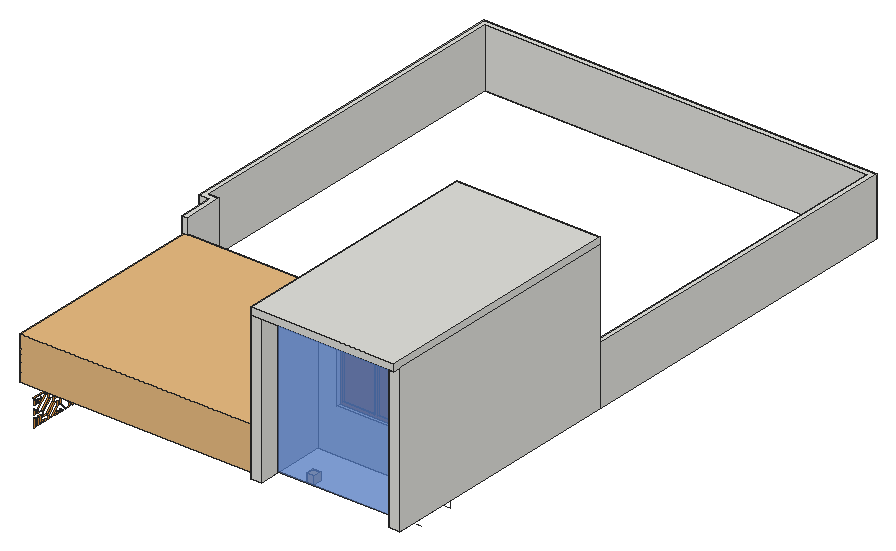
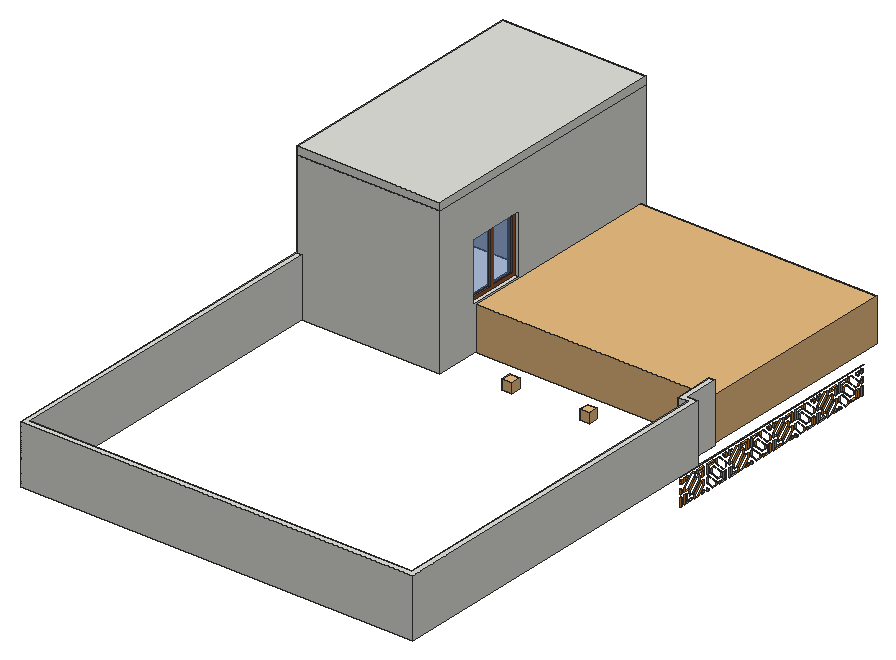
# SketchUp Ruby script. Lengths in inches.
U = 1.inch
M = Sketchup.active_model
def pt(a) = Geom::Point3d.new(a.map { |v| v * U })
def face(e, loops, mat)
  f = e.add_face(loops[0].map { |a| pt(a) })
  loops[1..].each { |l| e.add_face(l.map { |a| pt(a) }).erase! }
  f.material = f.back_material = mat if mat
  f
end
# faces: each face lists its corners as indices into pts; further lists are holes
def faces(e, pts, list, mat = nil) = list.each { |f| face(e, (f[0].is_a?(Array) ? f : [f]).map { |l| l.map { |i| pts[i] } }, mat) }
# xy, xz, yz: faces in a plane at the given z, y or x. An outline is a flat list of corners, or four numbers for a rectangle; further outlines are holes
def ring(l) = l.size == 4 ? [[l[0], l[1]], [l[2], l[1]], [l[2], l[3]], [l[0], l[3]]] : l.each_slice(2).to_a
def flat(e, list, mat, &to3) = list.each { |f| face(e, (f[0].is_a?(Array) ? f : [f]).map { |l| ring(l).map { |u, v| to3.(u, v) } }, mat) }
def xy(e, z, list, mat = nil) = flat(e, list, mat) { |x, y| [x, y, z] }
def xz(e, y, list, mat = nil) = flat(e, list, mat) { |x, z| [x, y, z] }
def yz(e, x, list, mat = nil) = flat(e, list, mat) { |y, z| [x, y, z] }
def lines(e, pts, list) = list.each { |a, b| e.add_line(pt(pts[a]), pt(pts[b])) }
# prism: a flat outline (further loops are holes) pulled along v
def prism(e, loops, v, mat = nil)
  f = face(e, loops, mat); d = Geom::Vector3d.new(v.map { |x| x * U })
  f.pushpull(f.normal.samedirection?(d) ? d.length : -d.length)
end
def box(e, o, s, mat = nil) = prism(e, [[o, [o[0] + s[0], o[1], o[2]], [o[0] + s[0], o[1] + s[1], o[2]], [o[0], o[1] + s[1], o[2]]]], [0, 0, s[2]], mat)
def at(x, y, z, deg = 0) = Geom::Transformation.translation(pt([x, y, z])) * Geom::Transformation.rotation(ORIGIN, Z_AXIS, deg.degrees)
def axes(o, x, y, z) = Geom::Transformation.new([*x, 0, *y, 0, *z, 0, *pt(o).to_a, 1])
def part(name) = M.definitions.add(name)
# library, detail: a bought-in or finely detailed component or shape, given as its bounding box
def library(name, o, s) = part(name).tap { |d| box(d.entities, o, s) }
def detail(e, o, s) = box(e.add_group.entities, o, s)
def put(e, d, t, mat = nil) = e.add_instance(d, t).tap { |i| i.material = mat if mat }
def group(e, t, mat = nil) = e.add_group.tap { |g| g.transformation = t; g.material = mat if mat }.entities
root = M.entities
M.materials.add("1056 AP 9903 Mellow Melon-N").color = [219, 142, 59]
M.materials.add("[Translucent Glass Blue]").color = [100, 149, 237]
M.materials["[Translucent Glass Blue]"].alpha = 0.5
M.materials.add("[Wood Cherry Original]").color = [152, 86, 42]
c1 = library("Sphere Light\#2",[-4,-4,-4],[8,8,8])
c2 = library("Sphere Light\#3",[-4,-4,-4],[8,8,8])
c3 = library("Sphere Light\#1",[-4.125,-4.125,-4.125],[8.25,8.25,8.25])
c4 = library("Sphere Light",[-3.2,-3.2,-3.2],[6.4,6.4,6.4])
c5 = part("Group10\#2")
xy(c5.entities,0,[[-21.5,-21.5,-1.25,21.5],[1.25,-21.5,21.5,21.5]])
c6 = part("Group9\#3")
prism(c6.entities,[[[24,-24,0],[-24,-24,0],[-24,24,0],[24,24,0]],[[-1.25,21.5,0],[-21.5,21.5,0],[-21.5,-21.5,0],[-1.25,-21.5,0]],[[1.25,-21.5,0],[21.5,-21.5,0],[21.5,21.5,0],[1.25,21.5,0]]],[0,0,2])
put(c6.entities,c5,at(0,0,1),"[Translucent Glass Blue]")
c7 = part("Group12\#2")
xy(c7.entities,0,[[-27.5,-21.5,-1.25,21.5],[1.25,-21.5,27.5,21.5]])
c8 = part("Group11\#3")
prism(c8.entities,[[[-30,24,0],[30,24,0],[30,-24,0],[-30,-24,0]],[[1.25,21.5,0],[1.25,-21.5,0],[27.5,-21.5,0],[27.5,21.5,0]],[[-1.25,-21.5,0],[-1.25,21.5,0],[-27.5,21.5,0],[-27.5,-21.5,0]]],[0,0,2])
put(c8.entities,c7,at(0,0,1))
c9 = part("Group53\#2")
prism(c9.entities,[[[11538.55,359.375,252],[11538.88,327.12,252],[11534.38,327.07,252],[11534.1,354.875,252],[11525.85,354.875,252],[11525.85,647.25,252],[11847.72,647.25,252],[11847.72,363.875,252],[11843.22,363.875,252],[11843.22,642.75,252],[11530.35,642.75,252],[11530.35,359.375,252]]],[0,0,48])
c10 = library("Glass Railing\#2",[-0.75,-168,0],[194.49,168.5,35.5])
xy(root,216.39,[[14.35,14.79,15.0625,15.84],[14.35,41.6875,15.0625,43.42],[14.35,47.3,15.0625,51.22],[14.35,53.82,15.0625,61.1875],[14.35,87.03,15.0625,88.76],
  [14.35,92.64,15.0625,96.56],[14.35,99.16,15.0625,106.53],[14.35,132.375,15.0625,134.11],[14.35,137.98,15.0625,141.91],[14.35,144.51,15.0625,151.875],
  [14.35,177.72,15.0625,179.45],[14.35,183.33,15.0625,187.25],[14.35,189.85,15.0625,197.22]],"1056 AP 9903 Mellow Melon-N")
xy(root,216.42,[[14.35,19.08,15.0625,25.95],[14.35,28.96,15.0625,32.8],[14.35,64.42,15.0625,71.3],[14.35,74.31,15.0625,78.15],[14.35,109.77,15.0625,116.64],
  [14.35,119.65,15.0625,123.49],[14.35,155.11,15.0625,161.99],[14.35,164.99,15.0625,168.84],[14.35,200.46,15.0625,201.3125]],"1056 AP 9903 Mellow Melon-N")
xy(root,217.72,[[14.35,21.23,15.0625,25.95],[14.35,66.57,15.0625,71.3],[14.35,111.92,15.0625,116.64],[14.35,157.26,15.0625,161.99]],"1056 AP 9903 Mellow Melon-N")
xy(root,218.1,[[14.35,41.25,15.0625,42.125],[14.35,53.82,15.0625,59.02],[14.35,86.6,15.0625,87.47],[14.35,99.16,15.0625,104.37],[14.35,131.94,15.0625,132.8125],
  [14.35,144.51,15.0625,149.71],[14.35,177.28,15.0625,178.16],[14.35,189.85,15.0625,195.05]],"1056 AP 9903 Mellow Melon-N")
xy(root,218.15,[[14.35,37.99,15.0625,38.41],[14.35,83.33,15.0625,83.76],[14.35,128.68,15.0625,129.1],[14.35,174.02,15.0625,174.45]],"1056 AP 9903 Mellow Melon-N")
xy(root,220.68,[[14.35,52.92,15.0625,55.99],[14.35,98.27,15.0625,101.33],[14.35,143.61,15.0625,146.68],[14.35,188.96,15.0625,192.02]],"1056 AP 9903 Mellow Melon-N")
xy(root,220.75,[[14.35,23.81,15.0625,27.21],[14.35,69.15,15.0625,72.56],[14.35,114.49,15.0625,117.9],[14.35,159.84,15.0625,163.24]],"1056 AP 9903 Mellow Melon-N")
xy(root,222.92,[[14.35,19.08,15.0625,21.23],[14.35,64.42,15.0625,66.57],[14.35,109.77,15.0625,111.92],[14.35,155.11,15.0625,157.26],[14.35,200.46,15.0625,201.3125]],"1056 AP 9903 Mellow Melon-N")
xy(root,223.26,[[14.35,14.79,15.0625,15.84],[14.35,59.02,15.0625,61.1875],[14.35,104.37,15.0625,106.53],[14.35,149.71,15.0625,151.875],[14.35,195.05,15.0625,197.22]],"1056 AP 9903 Mellow Melon-N")
xy(root,225.52,[[14.35,19.08,15.0625,22.06],[14.35,64.42,15.0625,67.4],[14.35,109.77,15.0625,112.75],[14.35,155.11,15.0625,158.09],[14.35,200.46,15.0625,201.3125]],"1056 AP 9903 Mellow Melon-N")
xy(root,225.84,[[14.35,14.79,15.0625,15.84],[14.35,41.6875,15.0625,44.32],[14.35,57.69,15.0625,61.1875],[14.35,87.03,15.0625,89.66],[14.35,103.04,15.0625,106.53],
  [14.35,132.375,15.0625,135],[14.35,148.38,15.0625,151.875],[14.35,177.72,15.0625,180.35],[14.35,193.72,15.0625,197.22]],"1056 AP 9903 Mellow Melon-N")
xy(root,225.95,[[14.35,35.87,15.0625,38.41],[14.35,81.21,15.0625,83.76],[14.35,126.55,15.0625,129.1],[14.35,171.9,15.0625,174.45]],"1056 AP 9903 Mellow Melon-N")
xy(root,228.55,[[14.35,36.7,15.0625,38.41],[14.35,82.04,15.0625,83.76],[14.35,127.38,15.0625,129.1],[14.35,172.73,15.0625,174.45]],"1056 AP 9903 Mellow Melon-N")
xy(root,228.84,[[14.35,41.6875,15.0625,42.99],[14.35,87.03,15.0625,88.33],[14.35,132.375,15.0625,133.67],[14.35,177.72,15.0625,179.02]],"1056 AP 9903 Mellow Melon-N")
xy(root,230.99,[[14.35,46.02,15.0625,49.09],[14.35,91.36,15.0625,94.43],[14.35,136.71,15.0625,139.77],[14.35,182.05,15.0625,185.12]],"1056 AP 9903 Mellow Melon-N")
xy(root,232.89,[[14.35,18.65,15.0625,19.5],[14.35,63.99,15.0625,64.84],[14.35,109.34,15.0625,110.1875],[14.35,154.68,15.0625,155.53],[14.35,200.03,15.0625,200.875]],"1056 AP 9903 Mellow Melon-N")
xy(root,233.14,[[14.35,14.97,15.0625,15.84],[14.35,60.3125,15.0625,61.1875],[14.35,105.66,15.0625,106.53],[14.35,151,15.0625,151.875],[14.35,196.34,15.0625,197.22]],"1056 AP 9903 Mellow Melon-N")
xy(root,233.57,[[14.35,42.99,15.0625,48.1875],[14.35,88.33,15.0625,93.53],[14.35,133.67,15.0625,138.875],[14.35,179.02,15.0625,184.22]],"1056 AP 9903 Mellow Melon-N")
xy(root,233.75,[[14.35,31.54,15.0625,36.7],[14.35,76.88,15.0625,82.04],[14.35,122.23,15.0625,127.38],[14.35,167.57,15.0625,172.73]],"1056 AP 9903 Mellow Melon-N")
xy(root,235.72,[[14.35,41.6875,15.0625,48.1875],[14.35,87.03,15.0625,93.53],[14.35,132.375,15.0625,138.875],[14.35,177.72,15.0625,184.22]],"1056 AP 9903 Mellow Melon-N")
xy(root,235.92,[[14.35,18.65,15.0625,21.66],[14.35,25.99,15.0625,28.96],[14.35,31.54,15.0625,38.41],[14.35,63.99,15.0625,67],[14.35,71.33,15.0625,74.31],
  [14.35,76.88,15.0625,83.76],[14.35,109.34,15.0625,112.35],[14.35,116.67,15.0625,119.65],[14.35,122.23,15.0625,129.1],[14.35,154.68,15.0625,157.6875],
  [14.35,162.02,15.0625,164.99],[14.35,167.57,15.0625,174.45],[14.35,200.03,15.0625,201.3125]],"1056 AP 9903 Mellow Melon-N")
xy(root,236.15,[[14.35,14.79,15.0625,15.84],[14.35,58.15,15.0625,61.1875],[14.35,103.5,15.0625,106.53],[14.35,148.84,15.0625,151.875],[14.35,194.1875,15.0625,197.22]],"1056 AP 9903 Mellow Melon-N")
xy(root,238.4375,[[14.35,13.79,15.0625,202.3125]],"1056 AP 9903 Mellow Melon-N")
xz(root,14.79,[[14.35,216.39,15.0625,223.26],[14.35,225.84,15.0625,229.87],[14.35,233.32,15.0625,236.15]],"1056 AP 9903 Mellow Melon-N")
xz(root,15.84,[[14.35,216.39,15.0625,223.26],[14.35,225.84,15.0625,228.8125],[14.35,233.14,15.0625,236.15]],"1056 AP 9903 Mellow Melon-N")
xz(root,18.65,[[14.35,232.89,15.0625,235.92]],"1056 AP 9903 Mellow Melon-N")
xz(root,19.08,[[14.35,216.42,15.0625,222.92]],"1056 AP 9903 Mellow Melon-N")
xz(root,21.23,[[14.35,217.72,15.0625,222.92]],"1056 AP 9903 Mellow Melon-N")
xz(root,21.66,[[14.35,235.04,15.0625,235.92]],"1056 AP 9903 Mellow Melon-N")
xz(root,23.81,[[14.35,220.75,15.0625,223.82]],"1056 AP 9903 Mellow Melon-N")
xz(root,25.95,[[14.35,216.42,15.0625,217.72]],"1056 AP 9903 Mellow Melon-N")
xz(root,28.96,[[14.35,216.42,15.0625,219.05],[14.35,232.42,15.0625,235.92]],"1056 AP 9903 Mellow Melon-N")
xz(root,31.54,[[14.35,233.75,15.0625,235.92]],"1056 AP 9903 Mellow Melon-N")
xz(root,34.12,[[14.35,227.66,15.0625,230.72]],"1056 AP 9903 Mellow Melon-N")
xz(root,36.7,[[14.35,215.99,15.0625,216.86],[14.35,228.55,15.0625,233.75]],"1056 AP 9903 Mellow Melon-N")
xz(root,38.41,[[14.35,216.42,15.0625,218.15],[14.35,222.03,15.0625,225.95],[14.35,228.55,15.0625,235.92]],"1056 AP 9903 Mellow Melon-N")
xz(root,41.6875,[[14.35,221.99,15.0625,225.84],[14.35,228.84,15.0625,235.72]],"1056 AP 9903 Mellow Melon-N")
xz(root,42.99,[[14.35,228.84,15.0625,233.57]],"1056 AP 9903 Mellow Melon-N")
xz(root,43.42,[[14.35,216.39,15.0625,216.81]],"1056 AP 9903 Mellow Melon-N")
xz(root,46.02,[[14.35,227.59,15.0625,230.99]],"1056 AP 9903 Mellow Melon-N")
xz(root,48.1875,[[14.35,233.57,15.0625,235.72]],"1056 AP 9903 Mellow Melon-N")
xz(root,50.79,[[14.35,232.74,15.0625,235.72]],"1056 AP 9903 Mellow Melon-N")
xz(root,51.22,[[14.35,216.39,15.0625,218.93]],"1056 AP 9903 Mellow Melon-N")
xz(root,53.82,[[14.35,216.39,15.0625,218.1]],"1056 AP 9903 Mellow Melon-N")
xz(root,58.15,[[14.35,235.3,15.0625,236.15]],"1056 AP 9903 Mellow Melon-N")
xz(root,59.02,[[14.35,218.1,15.0625,223.26]],"1056 AP 9903 Mellow Melon-N")
xz(root,61.1875,[[14.35,216.39,15.0625,223.26],[14.35,225.84,15.0625,228.8125],[14.35,233.14,15.0625,236.15]],"1056 AP 9903 Mellow Melon-N")
xz(root,63.99,[[14.35,232.89,15.0625,235.92]],"1056 AP 9903 Mellow Melon-N")
xz(root,64.42,[[14.35,216.42,15.0625,222.92]],"1056 AP 9903 Mellow Melon-N")
xz(root,66.57,[[14.35,217.72,15.0625,222.92]],"1056 AP 9903 Mellow Melon-N")
xz(root,67,[[14.35,235.04,15.0625,235.92]],"1056 AP 9903 Mellow Melon-N")
xz(root,69.15,[[14.35,220.75,15.0625,223.82]],"1056 AP 9903 Mellow Melon-N")
xz(root,71.3,[[14.35,216.42,15.0625,217.72]],"1056 AP 9903 Mellow Melon-N")
xz(root,74.31,[[14.35,216.42,15.0625,219.05],[14.35,232.42,15.0625,235.92]],"1056 AP 9903 Mellow Melon-N")
xz(root,76.88,[[14.35,233.75,15.0625,235.92]],"1056 AP 9903 Mellow Melon-N")
xz(root,79.46,[[14.35,227.66,15.0625,230.72]],"1056 AP 9903 Mellow Melon-N")
xz(root,82.04,[[14.35,215.99,15.0625,216.86],[14.35,228.55,15.0625,233.75]],"1056 AP 9903 Mellow Melon-N")
xz(root,83.76,[[14.35,216.42,15.0625,218.15],[14.35,222.03,15.0625,225.95],[14.35,228.55,15.0625,235.92]],"1056 AP 9903 Mellow Melon-N")
xz(root,87.03,[[14.35,221.99,15.0625,225.84],[14.35,228.84,15.0625,235.72]],"1056 AP 9903 Mellow Melon-N")
xz(root,88.33,[[14.35,228.84,15.0625,233.57]],"1056 AP 9903 Mellow Melon-N")
xz(root,88.76,[[14.35,216.39,15.0625,216.81]],"1056 AP 9903 Mellow Melon-N")
xz(root,91.36,[[14.35,227.59,15.0625,230.99]],"1056 AP 9903 Mellow Melon-N")
xz(root,93.53,[[14.35,233.57,15.0625,235.72]],"1056 AP 9903 Mellow Melon-N")
xz(root,96.13,[[14.35,232.74,15.0625,235.72]],"1056 AP 9903 Mellow Melon-N")
xz(root,96.56,[[14.35,216.39,15.0625,218.93]],"1056 AP 9903 Mellow Melon-N")
xz(root,99.16,[[14.35,216.39,15.0625,218.1]],"1056 AP 9903 Mellow Melon-N")
xz(root,103.5,[[14.35,235.3,15.0625,236.15]],"1056 AP 9903 Mellow Melon-N")
xz(root,104.37,[[14.35,218.1,15.0625,223.26]],"1056 AP 9903 Mellow Melon-N")
xz(root,106.53,[[14.35,216.39,15.0625,223.26],[14.35,225.84,15.0625,228.8125],[14.35,233.14,15.0625,236.15]],"1056 AP 9903 Mellow Melon-N")
xz(root,109.34,[[14.35,232.89,15.0625,235.92]],"1056 AP 9903 Mellow Melon-N")
xz(root,109.77,[[14.35,216.42,15.0625,222.92]],"1056 AP 9903 Mellow Melon-N")
xz(root,111.92,[[14.35,217.72,15.0625,222.92]],"1056 AP 9903 Mellow Melon-N")
xz(root,112.35,[[14.35,235.04,15.0625,235.92]],"1056 AP 9903 Mellow Melon-N")
xz(root,114.49,[[14.35,220.75,15.0625,223.82]],"1056 AP 9903 Mellow Melon-N")
xz(root,116.64,[[14.35,216.42,15.0625,217.72]],"1056 AP 9903 Mellow Melon-N")
xz(root,119.65,[[14.35,216.42,15.0625,219.05],[14.35,232.42,15.0625,235.92]],"1056 AP 9903 Mellow Melon-N")
xz(root,122.23,[[14.35,233.75,15.0625,235.92]],"1056 AP 9903 Mellow Melon-N")
xz(root,124.81,[[14.35,227.66,15.0625,230.72]],"1056 AP 9903 Mellow Melon-N")
xz(root,127.38,[[14.35,215.99,15.0625,216.86],[14.35,228.55,15.0625,233.75]],"1056 AP 9903 Mellow Melon-N")
xz(root,129.1,[[14.35,216.42,15.0625,218.15],[14.35,222.03,15.0625,225.95],[14.35,228.55,15.0625,235.92]],"1056 AP 9903 Mellow Melon-N")
xz(root,132.375,[[14.35,221.99,15.0625,225.84],[14.35,228.84,15.0625,235.72]],"1056 AP 9903 Mellow Melon-N")
xz(root,133.67,[[14.35,228.84,15.0625,233.57]],"1056 AP 9903 Mellow Melon-N")
xz(root,134.11,[[14.35,216.39,15.0625,216.81]],"1056 AP 9903 Mellow Melon-N")
xz(root,136.71,[[14.35,227.59,15.0625,230.99]],"1056 AP 9903 Mellow Melon-N")
xz(root,138.875,[[14.35,233.57,15.0625,235.72]],"1056 AP 9903 Mellow Melon-N")
xz(root,141.48,[[14.35,232.74,15.0625,235.72]],"1056 AP 9903 Mellow Melon-N")
xz(root,141.91,[[14.35,216.39,15.0625,218.93]],"1056 AP 9903 Mellow Melon-N")
xz(root,144.51,[[14.35,216.39,15.0625,218.1]],"1056 AP 9903 Mellow Melon-N")
xz(root,148.84,[[14.35,235.3,15.0625,236.15]],"1056 AP 9903 Mellow Melon-N")
xz(root,149.71,[[14.35,218.1,15.0625,223.26]],"1056 AP 9903 Mellow Melon-N")
xz(root,151.875,[[14.35,216.39,15.0625,223.26],[14.35,225.84,15.0625,228.8125],[14.35,233.14,15.0625,236.15]],"1056 AP 9903 Mellow Melon-N")
xz(root,154.68,[[14.35,232.89,15.0625,235.92]],"1056 AP 9903 Mellow Melon-N")
xz(root,155.11,[[14.35,216.42,15.0625,222.92]],"1056 AP 9903 Mellow Melon-N")
xz(root,157.26,[[14.35,217.72,15.0625,222.92]],"1056 AP 9903 Mellow Melon-N")
xz(root,157.6875,[[14.35,235.04,15.0625,235.92]],"1056 AP 9903 Mellow Melon-N")
xz(root,159.84,[[14.35,220.75,15.0625,223.82]],"1056 AP 9903 Mellow Melon-N")
xz(root,161.99,[[14.35,216.42,15.0625,217.72]],"1056 AP 9903 Mellow Melon-N")
xz(root,164.99,[[14.35,216.42,15.0625,219.05],[14.35,232.42,15.0625,235.92]],"1056 AP 9903 Mellow Melon-N")
xz(root,167.57,[[14.35,233.75,15.0625,235.92]],"1056 AP 9903 Mellow Melon-N")
xz(root,170.15,[[14.35,227.66,15.0625,230.72]],"1056 AP 9903 Mellow Melon-N")
xz(root,172.73,[[14.35,215.99,15.0625,216.86],[14.35,228.55,15.0625,233.75]],"1056 AP 9903 Mellow Melon-N")
xz(root,174.45,[[14.35,216.42,15.0625,218.15],[14.35,222.03,15.0625,225.95],[14.35,228.55,15.0625,235.92]],"1056 AP 9903 Mellow Melon-N")
xz(root,177.72,[[14.35,221.99,15.0625,225.84],[14.35,228.84,15.0625,235.72]],"1056 AP 9903 Mellow Melon-N")
xz(root,179.02,[[14.35,228.84,15.0625,233.57]],"1056 AP 9903 Mellow Melon-N")
xz(root,179.45,[[14.35,216.39,15.0625,216.81]],"1056 AP 9903 Mellow Melon-N")
xz(root,182.05,[[14.35,227.59,15.0625,230.99]],"1056 AP 9903 Mellow Melon-N")
xz(root,184.22,[[14.35,233.57,15.0625,235.72]],"1056 AP 9903 Mellow Melon-N")
xz(root,186.82,[[14.35,232.74,15.0625,235.72]],"1056 AP 9903 Mellow Melon-N")
xz(root,187.25,[[14.35,216.39,15.0625,218.93]],"1056 AP 9903 Mellow Melon-N")
xz(root,189.85,[[14.35,216.39,15.0625,218.1]],"1056 AP 9903 Mellow Melon-N")
xz(root,194.1875,[[14.35,235.3,15.0625,236.15]],"1056 AP 9903 Mellow Melon-N")
xz(root,195.05,[[14.35,218.1,15.0625,223.26]],"1056 AP 9903 Mellow Melon-N")
xz(root,197.22,[[14.35,216.39,15.0625,223.26],[14.35,225.84,15.0625,228.8125],[14.35,233.14,15.0625,236.15]],"1056 AP 9903 Mellow Melon-N")
xz(root,200.03,[[14.35,232.89,15.0625,235.92]],"1056 AP 9903 Mellow Melon-N")
xz(root,200.46,[[14.35,216.42,15.0625,222.92]],"1056 AP 9903 Mellow Melon-N")
xz(root,201.3125,[[14.35,216.42,15.0625,222.92],[14.35,225.52,15.0625,229.87],[14.35,233.32,15.0625,235.92]],"1056 AP 9903 Mellow Melon-N")
p = [[15.0625,36.7,215.99],[15.0625,38.41,216.42],[14.35,38.41,216.42],[14.35,36.7,215.99],[15.0625,82.04,215.99],[15.0625,83.76,216.42],
  [14.35,83.76,216.42],[14.35,82.04,215.99],[15.0625,127.38,215.99],[15.0625,129.1,216.42],[14.35,129.1,216.42],[14.35,127.38,215.99],
  [15.0625,172.73,215.99],[15.0625,174.45,216.42],[14.35,174.45,216.42],[14.35,172.73,215.99],[15.0625,32.8,216.42],[15.0625,38.41,222.03],
  [14.35,38.41,222.03],[14.35,32.8,216.42],[15.0625,41.25,218.1],[15.0625,41.6875,216.39],[14.35,41.6875,216.39],[14.35,41.25,218.1],
  [15.0625,41.6875,221.99],[15.0625,47.3,216.39],[14.35,47.3,216.39],[14.35,41.6875,221.99],[15.0625,78.15,216.42],[15.0625,83.76,222.03],
  [14.35,83.76,222.03],[14.35,78.15,216.42],[15.0625,86.6,218.1],[15.0625,87.03,216.39],[14.35,87.03,216.39],[14.35,86.6,218.1],
  [15.0625,87.03,221.99],[15.0625,92.64,216.39],[14.35,92.64,216.39],[14.35,87.03,221.99],[15.0625,123.49,216.42],[15.0625,129.1,222.03],
  [14.35,129.1,222.03],[14.35,123.49,216.42],[15.0625,131.94,218.1],[15.0625,132.375,216.39],[14.35,132.375,216.39],[14.35,131.94,218.1],
  [15.0625,132.375,221.99],[15.0625,137.98,216.39],[14.35,137.98,216.39],[14.35,132.375,221.99],[15.0625,168.84,216.42],[15.0625,174.45,222.03],
  [14.35,174.45,222.03],[14.35,168.84,216.42],[15.0625,177.28,218.1],[15.0625,177.72,216.39],[14.35,177.72,216.39],[14.35,177.28,218.1],
  [15.0625,177.72,221.99],[15.0625,183.33,216.39],[14.35,183.33,216.39],[14.35,177.72,221.99],[15.0625,43.42,216.81],[15.0625,42.125,218.1],
  [14.35,42.125,218.1],[14.35,43.42,216.81],[15.0625,88.76,216.81],[15.0625,87.47,218.1],[14.35,87.47,218.1],[14.35,88.76,216.81],
  [15.0625,134.11,216.81],[15.0625,132.8125,218.1],[14.35,132.8125,218.1],[14.35,134.11,216.81],[15.0625,179.45,216.81],[15.0625,178.16,218.1],
  [14.35,178.16,218.1],[14.35,179.45,216.81],[15.0625,37.99,218.15],[15.0625,36.7,216.86],[14.35,36.7,216.86],[14.35,37.99,218.15],
  [15.0625,83.33,218.15],[15.0625,82.04,216.86],[14.35,82.04,216.86],[14.35,83.33,218.15],[15.0625,128.68,218.15],[15.0625,127.38,216.86],
  [14.35,127.38,216.86],[14.35,128.68,218.15],[15.0625,174.02,218.15],[15.0625,172.73,216.86],[14.35,172.73,216.86],[14.35,174.02,218.15],
  [15.0625,51.22,218.93],[15.0625,44.32,225.84],[14.35,44.32,225.84],[14.35,51.22,218.93],[15.0625,96.56,218.93],[15.0625,89.66,225.84],
  [14.35,89.66,225.84],[14.35,96.56,218.93],[15.0625,141.91,218.93],[15.0625,135,225.84],[14.35,135,225.84],[14.35,141.91,218.93],
  [15.0625,187.25,218.93],[15.0625,180.35,225.84],[14.35,180.35,225.84],[14.35,187.25,218.93],[15.0625,35.87,225.95],[15.0625,28.96,219.05],
  [14.35,28.96,219.05],[14.35,35.87,225.95],[15.0625,81.21,225.95],[15.0625,74.31,219.05],[14.35,74.31,219.05],[14.35,81.21,225.95],
  [15.0625,126.55,225.95],[15.0625,119.65,219.05],[14.35,119.65,219.05],[14.35,126.55,225.95],[15.0625,171.9,225.95],[15.0625,164.99,219.05],
  [14.35,164.99,219.05],[14.35,171.9,225.95],[15.0625,46.02,227.59],[15.0625,52.92,220.68],[14.35,52.92,220.68],[14.35,46.02,227.59],
  [15.0625,55.99,220.68],[15.0625,56.42,223.66],[14.35,56.42,223.66],[14.35,55.99,220.68],[15.0625,91.36,227.59],[15.0625,98.27,220.68],
  [14.35,98.27,220.68],[14.35,91.36,227.59],[15.0625,101.33,220.68],[15.0625,101.76,223.66],[14.35,101.76,223.66],[14.35,101.33,220.68],
  [15.0625,136.71,227.59],[15.0625,143.61,220.68],[14.35,143.61,220.68],[14.35,136.71,227.59],[15.0625,146.68,220.68],[15.0625,147.1,223.66],
  [14.35,147.1,223.66],[14.35,146.68,220.68],[15.0625,182.05,227.59],[15.0625,188.96,220.68],[14.35,188.96,220.68],[14.35,182.05,227.59],
  [15.0625,192.02,220.68],[15.0625,192.45,223.66],[14.35,192.45,223.66],[14.35,192.02,220.68],[15.0625,27.21,220.75],[15.0625,34.12,227.66],
  [14.35,34.12,227.66],[14.35,27.21,220.75],[15.0625,72.56,220.75],[15.0625,79.46,227.66],[14.35,79.46,227.66],[14.35,72.56,220.75],
  [15.0625,117.9,220.75],[15.0625,124.81,227.66],[14.35,124.81,227.66],[14.35,117.9,220.75],[15.0625,163.24,220.75],[15.0625,170.15,227.66],
  [14.35,170.15,227.66],[14.35,163.24,220.75],[15.0625,49.09,230.99],[14.35,49.09,230.99],[15.0625,94.43,230.99],[14.35,94.43,230.99],
  [15.0625,139.77,230.99],[14.35,139.77,230.99],[15.0625,185.12,230.99],[14.35,185.12,230.99],[15.0625,31.14,231.15],[15.0625,23.81,223.82],
  [14.35,23.81,223.82],[14.35,31.14,231.15],[15.0625,76.48,231.15],[15.0625,69.15,223.82],[14.35,69.15,223.82],[14.35,76.48,231.15],
  [15.0625,121.83,231.15],[15.0625,114.49,223.82],[14.35,114.49,223.82],[14.35,121.83,231.15],[15.0625,167.17,231.15],[15.0625,159.84,223.82],
  [14.35,159.84,223.82],[14.35,167.17,231.15],[15.0625,18.65,228.58],[15.0625,19.08,225.52],[14.35,19.08,225.52],[14.35,18.65,228.58],
  [15.0625,22.06,225.52],[15.0625,28.96,232.42],[14.35,28.96,232.42],[14.35,22.06,225.52],[15.0625,63.99,228.58],[15.0625,64.42,225.52],
  [14.35,64.42,225.52],[14.35,63.99,228.58],[15.0625,67.4,225.52],[15.0625,74.31,232.42],[14.35,74.31,232.42],[14.35,67.4,225.52],
  [15.0625,109.33,228.58],[15.0625,109.77,225.52],[14.35,109.77,225.52],[14.35,109.33,228.58],[15.0625,112.75,225.52],[15.0625,119.65,232.42],
  [14.35,119.65,232.42],[14.35,112.75,225.52],[15.0625,154.68,228.58],[15.0625,155.11,225.52],[14.35,155.11,225.52],[14.35,154.68,228.58],
  [15.0625,158.09,225.52],[15.0625,164.99,232.42],[14.35,164.99,232.42],[14.35,158.09,225.52],[15.0625,200.02,228.58],[15.0625,200.46,225.52],
  [14.35,200.46,225.52],[14.35,200.02,228.58],[15.0625,50.79,232.74],[15.0625,57.69,225.84],[14.35,57.69,225.84],[14.35,50.79,232.74],
  [15.0625,96.13,232.74],[15.0625,103.04,225.84],[14.35,103.04,225.84],[14.35,96.13,232.74],[15.0625,141.48,232.74],[15.0625,148.38,225.84],
  [14.35,148.38,225.84],[14.35,141.48,232.74],[15.0625,186.82,232.74],[15.0625,193.72,225.84],[14.35,193.72,225.84],[14.35,186.82,232.74],
  [15.0625,25.99,235.92],[14.35,25.99,235.92],[15.0625,71.33,235.92],[14.35,71.33,235.92],[15.0625,116.67,235.92],[14.35,116.67,235.92],
  [15.0625,162.02,235.92],[14.35,162.02,235.92],[15.0625,201.3125,229.87],[14.35,201.3125,229.87],[15.0625,15.84,228.8125],[15.0625,14.79,229.87],
  [14.35,14.79,229.87],[14.35,15.84,228.8125],[15.0625,61.1875,228.8125],[15.0625,53.85,236.15],[14.35,53.85,236.15],[14.35,61.1875,228.8125],
  [15.0625,106.53,228.8125],[15.0625,99.19,236.15],[14.35,99.19,236.15],[14.35,106.53,228.8125],[15.0625,151.875,228.8125],[15.0625,144.54,236.15],
  [14.35,144.54,236.15],[14.35,151.875,228.8125],[15.0625,197.22,228.8125],[15.0625,189.88,236.15],[14.35,189.88,236.15],[14.35,197.22,228.8125],
  [15.0625,34.12,230.72],[14.35,34.12,230.72],[15.0625,79.46,230.72],[14.35,79.46,230.72],[15.0625,124.81,230.72],[14.35,124.81,230.72],
  [15.0625,170.15,230.72],[14.35,170.15,230.72],[15.0625,19.5,232.89],[15.0625,21.66,235.04],[14.35,21.66,235.04],[14.35,19.5,232.89],
  [15.0625,64.84,232.89],[15.0625,67,235.04],[14.35,67,235.04],[14.35,64.84,232.89],[15.0625,110.1875,232.89],[15.0625,112.35,235.04],
  [14.35,112.35,235.04],[14.35,110.1875,232.89],[15.0625,155.53,232.89],[15.0625,157.6875,235.04],[14.35,157.6875,235.04],[14.35,155.53,232.89],
  [15.0625,200.875,232.89],[15.0625,201.3125,233.32],[14.35,201.3125,233.32],[14.35,200.875,232.89],[15.0625,14.79,233.32],[15.0625,14.97,233.14],
  [14.35,14.97,233.14],[14.35,14.79,233.32],[15.0625,58.15,235.3],[15.0625,60.3125,233.14],[14.35,60.3125,233.14],[14.35,58.15,235.3],
  [15.0625,103.5,235.3],[15.0625,105.66,233.14],[14.35,105.66,233.14],[14.35,103.5,235.3],[15.0625,148.84,235.3],[15.0625,151,233.14],
  [14.35,151,233.14],[14.35,148.84,235.3],[15.0625,194.1875,235.3],[15.0625,196.34,233.14],[14.35,196.34,233.14],[14.35,194.1875,235.3],
  [15.0625,50.79,235.72],[14.35,50.79,235.72],[15.0625,96.13,235.72],[14.35,96.13,235.72],[15.0625,141.48,235.72],[14.35,141.48,235.72],
  [15.0625,186.82,235.72],[14.35,186.82,235.72],[291.22,58.1875,252],[321.875,58.1875,252],[321.875,58.1875,246],[291.22,58.1875,246],
  [317.35,28.25,246],[321.875,28.25,246],[15.0625,202.3125,238.4375],[15.0625,13.79,238.4375]]
faces(root,p,[[0,1,2,3],[4,5,6,7],[8,9,10,11],[12,13,14,15],[16,17,18,19],[20,21,22,23],[24,25,26,27],[28,29,30,31],
  [32,33,34,35],[36,37,38,39],[40,41,42,43],[44,45,46,47],[48,49,50,51],[52,53,54,55],[56,57,58,59],[60,61,62,63],
  [64,65,66,67],[68,69,70,71],[72,73,74,75],[76,77,78,79],[80,81,82,83],[84,85,86,87],[88,89,90,91],[92,93,94,95],
  [96,97,98,99],[100,101,102,103],[104,105,106,107],[108,109,110,111],[112,113,114,115],[116,117,118,119],[120,121,122,123],[124,125,126,127],
  [128,129,130,131],[132,133,134,135],[136,137,138,139],[140,141,142,143],[144,145,146,147],[148,149,150,151],[152,153,154,155],[156,157,158,159],
  [160,161,162,163],[164,165,166,167],[168,169,170,171],[172,173,174,175],[133,176,177,134],[141,178,179,142],[149,180,181,150],[157,182,183,158],
  [184,185,186,187],[188,189,190,191],[192,193,194,195],[196,197,198,199],[200,201,202,203],[204,205,206,207],[208,209,210,211],[212,213,214,215],
  [216,217,218,219],[220,221,222,223],[224,225,226,227],[228,229,230,231],[232,233,234,235],[236,237,238,239],[240,241,242,243],[244,245,246,247],
  [248,249,250,251],[252,200,203,253],[254,208,211,255],[256,216,219,257],[258,224,227,259],[260,232,235,261],[262,263,264,265],[266,267,268,269],
  [270,271,272,273],[274,275,276,277],[278,279,280,281],[282,184,187,283],[284,188,191,285],[286,192,195,287],[288,196,199,289],[290,291,292,293],
  [294,295,296,297],[298,299,300,301],[302,303,304,305],[306,307,308,309],[310,311,312,313],[314,315,316,317],[318,319,320,321],[322,323,324,325],
  [326,327,328,329],[267,330,331,268],[271,332,333,272],[275,334,335,276],[279,336,337,280]],"1056 AP 9903 Mellow Melon-N")
lines(root,p,[[338,339],[339,340],[340,341],[342,343],[344,345]])
put(root,c1,at(39.1,135.28,246))
put(root,c2,at(39.1,186.08,246))
put(root,c3,at(39.1,84.48,247))
put(root,c2,at(102.67,186.08,247))
put(root,c2,at(166.24,186.08,247))
put(root,c2,at(229.8125,186.08,247))
put(root,c2,at(229.8125,135.28,247))
put(root,c2,at(229.8125,84.48,247))
put(root,c2,at(166.24,84.48,247))
put(root,c2,at(102.67,84.48,247))
put(root,c2,at(39.1,84.48,247))
put(root,c2,at(166.3125,135.28,247))
put(root,c2,at(102.8125,135.28,247))
put(root,c2,at(39.3125,135.28,247))
put(root,c4,at(39.1,33.68,247))
put(root,c4,at(102.35,33.68,247))
put(root,c4,at(165.6,33.68,247))
put(root,c4,at(228.85,33.68,247))
g1 = group(root,at(21.875,58.1875,252))
xy(g1,0,[[[182.15,-58.1875,182.15,153.125,300,153.125,300,-52.5625,291,-52.5625,291,0,191.15,0,191.15,-58.1875],[191.15,9,291,144.125]]])
xy(g1,36,[[206.15,0,266.15,4.5],[206.15,4.5,266.15,9],[182.15,72.125,186.65,120.125],[186.65,72.125,191.15,120.125]])
xy(g1,84,[[206.15,0,266.15,4.5],[206.15,4.5,266.15,9],[182.15,72.125,186.65,120.125],[186.65,72.125,191.15,120.125]])
xy(g1,120,[[[182.15,-58.1875,191.15,-58.1875,191.15,0,291,0,291,-52.5625,300,-52.5625,300,153.125,182.15,153.125],[191.15,9,291,144.125]]])
xz(g1,-58.1875,[[182.15,0,191.15,120]])
xz(g1,-52.5625,[[291,0,300,120]])
xz(g1,0,[[[191.15,0,291,120],[206.15,36,266.15,84]]])
xz(g1,9,[[[191.15,0,291,120],[206.15,36,266.15,84]]])
xz(g1,72.125,[[182.15,36,186.65,84],[186.65,36,191.15,84]])
xz(g1,120.125,[[182.15,36,186.65,84],[186.65,36,191.15,84]])
xz(g1,144.125,[[191.15,0,291,120]])
xz(g1,153.125,[[182.15,0,300,120]])
yz(g1,182.15,[[[-58.1875,0,153.125,120],[72.125,36,120.125,84]]])
yz(g1,191.15,[[-58.1875,0,0,120],[[9,0,144.125,120],[72.125,36,120.125,84]]])
yz(g1,206.15,[[0,36,4.5,84],[4.5,36,9,84]])
yz(g1,266.15,[[0,36,4.5,84],[4.5,36,9,84]])
yz(g1,291,[[-52.5625,0,0,120],[9,0,144.125,120]])
yz(g1,300,[[-52.5625,0,153.125,120]])
p = [[291,144.125,0],[291,153.125,0]]
lines(g1,p,[[0,1]])
put(g1,c6,axes([187.65,96.125,60],[0,-1,0],[0,0,1],[-1,0,0]),"[Wood Cherry Original]")
put(g1,c8,axes([236.15,3.5,60],[-1,0,0],[0,0,1],[0,1,0]),"[Wood Cherry Original]")
put(root,c9,at(-11525.85,-152.5625,0))
g2 = group(root,at(213.02,12.25,252))
box(g2,[0,4.9375,0],[99.85,1.1875,120],"[Translucent Glass Blue]")
p = [[0,0,120],[0,4.9375,120],[99.85,0,120],[99.85,4.9375,120],[99.85,0,0],[99.85,4.9375,0],
  [0,0,0],[0,4.9375,0]]
lines(g2,p,[[0,1],[2,3],[4,5],[6,7]])
put(root,c10,at(10.78,174.53,252))
g3 = group(root,at(204.02,58.1875,372))
box(g3,[0,-58.1875,0],[117.85,211.3125,6])
